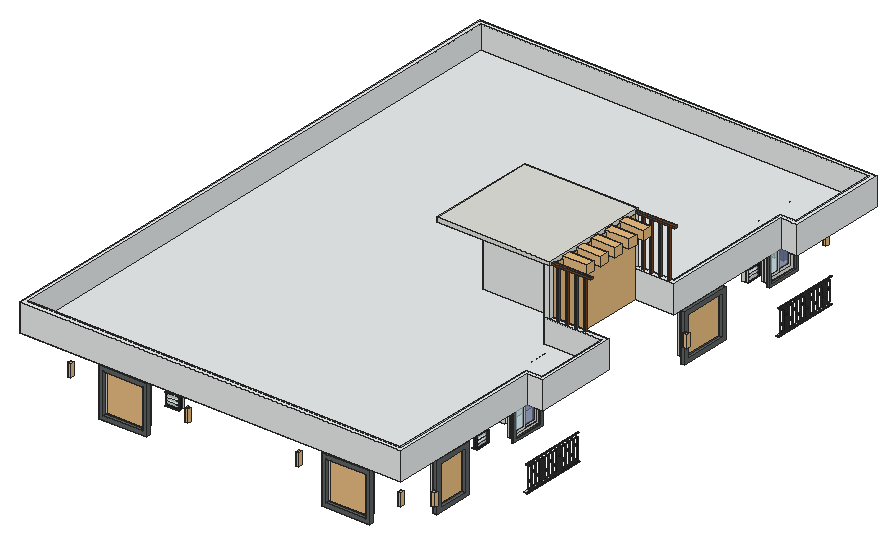
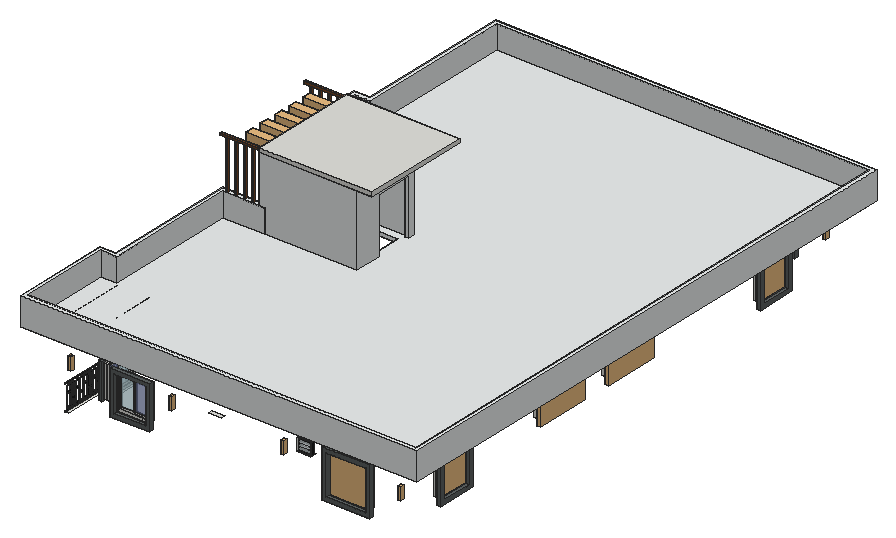
# SketchUp Ruby script. Lengths in inches.
U = 1.inch
M = Sketchup.active_model
def pt(a) = Geom::Point3d.new(a.map { |v| v * U })
def face(e, loops, mat)
  f = e.add_face(loops[0].map { |a| pt(a) })
  loops[1..].each { |l| e.add_face(l.map { |a| pt(a) }).erase! }
  f.material = f.back_material = mat if mat
  f
end
# faces: each face lists its corners as indices into pts; further lists are holes
def faces(e, pts, list, mat = nil) = list.each { |f| face(e, (f[0].is_a?(Array) ? f : [f]).map { |l| l.map { |i| pts[i] } }, mat) }
# xy, xz, yz: faces in a plane at the given z, y or x. An outline is a flat list of corners, or four numbers for a rectangle; further outlines are holes
def ring(l) = l.size == 4 ? [[l[0], l[1]], [l[2], l[1]], [l[2], l[3]], [l[0], l[3]]] : l.each_slice(2).to_a
def flat(e, list, mat, &to3) = list.each { |f| face(e, (f[0].is_a?(Array) ? f : [f]).map { |l| ring(l).map { |u, v| to3.(u, v) } }, mat) }
def xy(e, z, list, mat = nil) = flat(e, list, mat) { |x, y| [x, y, z] }
def xz(e, y, list, mat = nil) = flat(e, list, mat) { |x, z| [x, y, z] }
def yz(e, x, list, mat = nil) = flat(e, list, mat) { |y, z| [x, y, z] }
def lines(e, pts, list) = list.each { |a, b| e.add_line(pt(pts[a]), pt(pts[b])) }
# prism: a flat outline (further loops are holes) pulled along v
def prism(e, loops, v, mat = nil)
  f = face(e, loops, mat); d = Geom::Vector3d.new(v.map { |x| x * U })
  f.pushpull(f.normal.samedirection?(d) ? d.length : -d.length)
end
def box(e, o, s, mat = nil) = prism(e, [[o, [o[0] + s[0], o[1], o[2]], [o[0] + s[0], o[1] + s[1], o[2]], [o[0], o[1] + s[1], o[2]]]], [0, 0, s[2]], mat)
def at(x, y, z, deg = 0) = Geom::Transformation.translation(pt([x, y, z])) * Geom::Transformation.rotation(ORIGIN, Z_AXIS, deg.degrees)
def axes(o, x, y, z) = Geom::Transformation.new([*x, 0, *y, 0, *z, 0, *pt(o).to_a, 1])
def part(name) = M.definitions.add(name)
# library, detail: a bought-in or finely detailed component or shape, given as its bounding box
def library(name, o, s) = part(name).tap { |d| box(d.entities, o, s) }
def detail(e, o, s) = box(e.add_group.entities, o, s)
def put(e, d, t, mat = nil) = e.add_instance(d, t).tap { |i| i.material = mat if mat }
def group(e, t, mat = nil) = e.add_group.tap { |g| g.transformation = t; g.material = mat if mat }.entities
root = M.entities
M.materials.add("1487 AP 8286 CHARCOAL SHADOW").color = [94, 99, 99]
M.materials.add("[3P0081_White-City]").color = [235, 238, 238]
M.materials.add("[Color M08]").color = [30, 30, 30]
M.materials.add("[Color_008]1").color = [30, 30, 30]
M.materials.add("[Translucent Glass Safety]").color = [218, 227, 229]
M.materials["[Translucent Glass Safety]"].alpha = 0.5
M.materials.add("[Translucent_Glass_Safety]").color = [204, 235, 244]
M.materials["[Translucent_Glass_Safety]"].alpha = 0.5
M.materials.add("[Translucent_Glass_Sky_Reflection]").color = [125, 138, 183]
M.materials["[Translucent_Glass_Sky_Reflection]"].alpha = 0.52
M.materials.add("[Wood Veneer 01]").color = [120, 70, 37]
c1 = library("porta 4",[0.2,-5.42,1.33],[46.55,4.72,83.21])
c2 = part("Group\#70")
prism(c2.entities,[[[4.13,0,3.9375],[7.875,0,3.9375],[7.875,0,13.78],[4.13,0,13.78],[4.13,0,15.75],[7.875,0,15.75],[7.875,0,35.43],[4.13,0,35.43],[4.13,0,39.37],[3.74,0,39.37],[3.74,0,35.43],[0,0,35.43],[0,0,15.75],[3.74,0,15.75],[3.74,0,13.78],[0,0,13.78],[0,0,3.9375],[3.74,0,3.9375],[3.74,0,0],[4.13,0,0]],[[0.39,0,16.14],[0.39,0,35.04],[7.48,0,35.04],[7.48,0,16.14]],[[7.48,0,4.33],[0.39,0,4.33],[0.39,0,13.39],[7.48,0,13.39]]],[0,0.39,0],"[Color M08]")
c3 = part("Group\#69")
prism(c3.entities,[[[3.74,0,35.43],[0,0,35.43],[0,0,25.59],[3.74,0,25.59],[3.74,0,23.62],[0,0,23.62],[0,0,3.9375],[3.74,0,3.9375],[3.74,0,0],[4.13,0,0],[4.13,0,3.9375],[7.875,0,3.9375],[7.875,0,23.62],[4.13,0,23.62],[4.13,0,25.59],[7.875,0,25.59],[7.875,0,35.43],[4.13,0,35.43],[4.13,0,39.37],[3.74,0,39.37]],[[7.48,0,23.23],[7.48,0,4.33],[0.39,0,4.33],[0.39,0,23.23]],[[0.39,0,35.04],[7.48,0,35.04],[7.48,0,25.98],[0.39,0,25.98]]],[0,0.39,0],"[Color M08]")
c4 = part("Group\#71")
put(c4.entities,c2,at(0,0,0))
put(c4.entities,c3,at(9.84,0,0))
c5 = part("Group\#79")
g1 = group(c5.entities,at(0,0,0))
box(g1,[0,-2.09,0],[1.97,122.29,0.79],"[Color M08]")
put(c5.entities,c4,axes([0.79,40.35,0.79],[0,1,0],[1,0,0],[0,0,1]))
put(c5.entities,c4,axes([0.79,79.72,0.79],[0,1,0],[1,0,0],[0,0,1]))
put(c5.entities,c4,axes([0.79,60.04,0.79],[0,1,0],[1,0,0],[0,0,1]))
put(c5.entities,c4,axes([0.79,99.41,0.79],[0,1,0],[1,0,0],[0,0,1]))
g2 = group(c5.entities,at(0,0,40.16))
box(g2,[0,-2.09,0],[1.97,122.29,0.79],"[Color M08]")
put(c5.entities,c4,axes([0.79,20.67,0.79],[0,1,0],[1,0,0],[0,0,1]))
put(c5.entities,c4,axes([0.79,0.98,0.79],[0,1,0],[1,0,0],[0,0,1]))
c6 = part("14")
prism(c6.entities,[[[0,60,66],[0,0,66],[0,0,0],[0,60,0]],[[0,54,6],[0,6,6],[0,6,60],[0,54,60]]],[-6,0,0])
c7 = library("15",[-6,0,0],[6,84,66])
c8 = part("17")
prism(c8.entities,[[[0,0,0],[0,0,72],[72,0,72],[72,0,0]],[[6,0,6],[66,0,6],[66,0,66],[6,0,66]]],[0,-6,0])
c9 = library("Group\#98",[0,-5.45,0],[91.05,108.7,8])
c10 = part("Two-panel window")
xy(c10.entities,0,[[0,0,4.33,55.51]])
xy(c10.entities,2.76,[[0,2.76,2,2.76,2,27.76,0.82,27.76,0.82,52.76,0,52.76],[3.15,2.76,4.33,2.76,4.33,52.76,2.36,52.76,2.36,27.76,3.15,27.76],[0.82,27.76,2.36,52.76]])
xy(c10.entities,4.72,[[2,4.72,2.4,26.38],[2.76,4.72,3.15,26.38],[0.82,29.13,1.22,50.79],[1.97,29.13,2.36,50.79]])
xy(c10.entities,36.61,[[2,4.72,2.4,26.38],[2.76,4.72,3.15,26.38],[0.82,29.13,1.22,50.79],[1.97,29.13,2.36,50.79]])
xy(c10.entities,38.58,[[0,2.76,2,27.76],[3.15,2.76,4.33,27.76],[0,27.76,0.82,52.76],[0.82,27.76,2.36,52.76],[2.36,27.76,4.33,52.76]])
xy(c10.entities,41.34,[[0,0,4.33,55.51]])
xz(c10.entities,0,[[0,0,4.33,41.34]])
xz(c10.entities,2.76,[[0,2.76,2,38.58],[3.15,2.76,4.33,38.58]])
xz(c10.entities,4.72,[[2,4.72,2.4,36.61],[2.76,4.72,3.15,36.61]])
xz(c10.entities,26.38,[[2,4.72,2.4,36.61],[2.76,4.72,3.15,36.61]])
xz(c10.entities,27.76,[[0.82,2.76,2,38.58],[2,2.76,2.36,38.58],[2.36,2.76,3.15,38.58]])
xz(c10.entities,29.13,[[0.82,4.72,1.22,36.61],[1.97,4.72,2.36,36.61]])
xz(c10.entities,50.79,[[0.82,4.72,1.22,36.61],[1.97,4.72,2.36,36.61]])
xz(c10.entities,52.76,[[0,2.76,0.82,38.58],[0.82,2.76,2.36,38.58],[2.36,2.76,4.33,38.58]])
xz(c10.entities,55.51,[[0,0,4.33,41.34]])
yz(c10.entities,0,[[[0,0,55.51,41.34],[2.76,2.76,52.76,38.58]]])
yz(c10.entities,0.82,[[[27.76,2.76,52.76,38.58],[29.13,4.72,50.79,36.61]]])
yz(c10.entities,1.22,[[29.13,4.72,50.79,36.61]],"[Translucent_Glass_Sky_Reflection]")
yz(c10.entities,1.97,[[29.13,4.72,50.79,36.61]],"[Translucent_Glass_Sky_Reflection]")
yz(c10.entities,2,[[[2.76,2.76,27.76,38.58],[4.72,4.72,26.38,36.61]]])
yz(c10.entities,2.36,[[[27.76,2.76,52.76,38.58],[29.13,4.72,50.79,36.61]]])
yz(c10.entities,2.4,[[4.72,4.72,26.38,36.61]],"[Translucent_Glass_Safety]")
yz(c10.entities,2.76,[[4.72,4.72,26.38,36.61]],"[Translucent_Glass_Safety]")
yz(c10.entities,3.15,[[[2.76,2.76,27.76,38.58],[4.72,4.72,26.38,36.61]]])
yz(c10.entities,4.33,[[[0,0,55.51,41.34],[2.76,2.76,52.76,38.58]]])
c11 = library("Group\#50",[0,-5.45,0],[91.05,108.7,8])
c12 = library("Group\#36",[0,-5.45,0],[91.05,108.7,8])
c13 = library("Group\#28",[0.125,0,-2.28],[4,104,84.28])
c14 = library("WALL LIGHT 69",[4.19,4.05,-9.73],[4.61,5.7,19.03])
c15 = part("Group\#40")
box(c15.entities,[0,0.25,0],[21,0.25,6],"[Translucent Glass Safety]")
c16 = part("tingkap keping toilet")
g3 = group(c16.entities,at(-23.5,-2,0),"[Color_008]1")
prism(g3,[[[47,0,57],[22.5,0,57],[22.5,0,41.8],[47,0,41.8]],[[24.5,0,43.3],[24.5,0,55.5],[45.5,0,55.5],[45.5,0,43.3]]],[0,4,0])
g4 = group(c16.entities,at(1,-2,47))
put(g4,c15,axes([0,3.73,3.53],[1,0,0],[0,0.757,0.65342],[0,-0.65342,0.757]))
put(g4,c15,axes([0,3.73,-0.17],[1,0,0],[0,0.757,0.65342],[0,-0.65342,0.757]))
put(g4,c15,axes([0,3.73,-3.87],[1,0,0],[0,0.757,0.65342],[0,-0.65342,0.757]))
c17 = library("Floor panel",[0,13.98,-0.38],[148.62,177.51,16.92])
c18 = library("Group\#130",[0,6,-42],[1.25,152,114])
c19 = library("20",[0,-4.6875,-10.69],[37.375,13.375,13.69])
xy(root,266,[[682.5,564.97,688.5,663.97],[553.5,678.97,562.5,738.97],[679.5,1044.97,685.5,1143.97]])
xy(root,294,[[649.5,897.97,658.5,963.97]])
xy(root,300,[[218,357.97,278,366.97],[554.5,357.97,614.5,366.97],[171,426.87,180,474.87],[652.5,426.87,661.5,474.87],[493.5,600.97,513.5,606.97],
  [622.5,609.97,631.5,657.97],[198,654.97,207,726.97],[198,783.97,207,855.97],[171,1029.97,180,1077.97],[493.5,1080.97,513.5,1086.97],
  [622.5,1089.97,631.5,1137.97],[218,1143.97,278,1152.97],[550.5,1143.97,598.5,1152.97]])
xy(root,342,[[306,357.97,327.5,366.97],[652.5,504.97,661.5,526.53],[382.75,726.97,404.25,735.97],[382.75,774.97,404.25,783.97],[649.5,1017.47,658.5,1038.97],
  [306,1143.97,327.5,1152.97]])
xy(root,348,[[309,453.97,333,459.97],[360,462.97,366,492.97],[507,498.97,539,504.97],[553.5,498.97,583.5,504.97],[622.5,567.97,631.5,597.97],
  [622.5,609.97,631.5,657.97],[321,624.97,357,630.97],[433.5,663.97,472.5,672.97],[363,666.97,369,690.97],[363,819.97,369,843.97],
  [433.5,837.97,472.5,846.97],[321,879.97,357,885.97],[504,978.97,536,984.97],[550.5,978.97,580.5,984.97],[360,1017.47,366,1047.47],
  [622.5,1047.97,631.5,1077.97],[309,1050.97,333,1056.97],[622.5,1089.97,631.5,1137.97]])
xy(root,354,[[386.25,387.97,470.25,396.97],[171,426.87,180,474.87],[198,530.97,207,614.97],[198,654.97,207,726.97],[198,783.97,207,855.97],
  [649.5,897.97,658.5,963.97],[198,903.97,207,987.97],[171,1029.97,180,1077.97],[386.25,1113.97,470.25,1122.97],[550.5,1143.97,598.5,1152.97]])
xy(root,360,[[218,357.97,278,366.97],[306,357.97,327.5,366.97],[554.5,357.97,614.5,366.97],[652.5,426.87,661.5,474.87],[652.5,504.97,661.5,526.53],
  [382.75,726.97,404.25,735.97],[382.75,774.97,404.25,783.97],[649.5,1017.47,658.5,1038.97],[218,1143.97,278,1152.97],[306,1143.97,327.5,1152.97]])
xy(root,390,[[[144,357.97,366,357.97,366,387.97,490.5,387.97,490.5,357.97,688.5,357.97,688.5,408.97,661.5,408.97,661.5,529,688.5,529,688.5,535,661.5,535,661.5,558.97,688.5,558.97,688.5,564.97,631.5,564.97,631.5,663.97,688.5,663.97,688.5,672.97,631.5,672.97,631.5,763.97,622.5,763.97,622.5,753.97,553.5,753.97,553.5,738.97,562.5,738.97,562.5,744.97,622.5,744.97,622.5,672.97,562.5,672.97,562.5,678.97,553.5,678.97,553.5,672.97,430.5,672.97,430.5,837.97,622.5,837.97,622.5,827.97,631.5,827.97,631.5,837.97,685.5,837.97,685.5,888.97,658.5,888.97,658.5,1009,685.5,1009,685.5,1015,658.5,1015,658.5,1038.97,649.5,1038.97,649.5,984.97,544.5,984.97,544.5,1038.97,685.5,1038.97,685.5,1044.97,631.5,1044.97,631.5,1143.97,685.5,1143.97,685.5,1152.97,487.5,1152.97,487.5,1122.97,366,1122.97,366,1152.97,144,1152.97,144,1101.97,171,1101.97,171,1005.97,198,1005.97,198,504.97,171,504.97,171,408.97,144,408.97],[366,396.97,366,504.97,207,504.97,207,624.97,427.5,624.97,427.5,663.97,487.5,663.97,487.5,572.47,421.5,572.47,421.5,537.97,427.5,537.97,427.5,566.47,487.5,566.47,487.5,537.97,493.5,537.97,493.5,663.97,622.5,663.97,622.5,564.97,541.5,564.97,541.5,504.97,490.5,504.97,490.5,396.97],[427.5,846.97,427.5,885.97,207,885.97,207,1005.97,366,1005.97,366,1113.97,487.5,1113.97,487.5,1080.97,493.5,1080.97,493.5,1143.97,622.5,1143.97,622.5,1044.97,487.5,1044.97,487.5,1014.97,493.5,1014.97,493.5,1038.97,538.5,1038.97,538.5,984.97,487.5,984.97,487.5,944.47,427.5,944.47,427.5,972.97,421.5,972.97,421.5,938.47,487.5,938.47,487.5,846.97],[496.5,366.97,496.5,495.97,504.5,495.97,504.5,498.97,617.5,498.97,617.5,495.97,631.5,495.97,631.5,498.97,652.5,498.97,652.5,399.97,679.5,399.97,679.5,366.97],[493.5,846.97,493.5,975.97,501.5,975.97,501.5,978.97,617.5,978.97,617.5,975.97,631.5,975.97,631.5,978.97,649.5,978.97,649.5,879.97,676.5,879.97,676.5,846.97],[207,630.97,207,750.97,372,750.97,372,774.97,421.5,774.97,421.5,735.97,372,735.97,372,750.97,363,750.97,363,630.97],[180,1011.97,180,1110.97,153,1110.97,153,1143.97,300,1143.97,300,1050.97,360,1050.97,360,1014.97,352,1014.97,352,1011.97],[153,366.97,153,399.97,180,399.97,180,498.97,352,498.97,352,495.97,360,495.97,360,459.97,300,459.97,300,366.97],[207,759.97,363,879.97],[547.5,504.97,652.5,558.97],[369,783.97,421.5,879.97],[369,630.97,421.5,726.97],[306,366.97,360,453.97],[306,1056.97,360,1143.97]]])
xz(root,426.87,[[171,300,180,354],[652.5,300,661.5,360]])
xz(root,474.87,[[171,300,180,354],[652.5,300,661.5,360]])
xz(root,526.53,[[652.5,342,661.5,360]])
xz(root,609.97,[[622.5,300,631.5,348]])
xz(root,654.97,[[198,300,207,354]])
xz(root,657.97,[[622.5,300,631.5,348]])
xz(root,678.97,[[553.5,266,562.5,390]])
xz(root,726.97,[[198,300,207,354]])
xz(root,738.97,[[553.5,266,562.5,390]])
xz(root,783.97,[[198,300,207,354]])
xz(root,855.97,[[198,300,207,354]])
xz(root,897.97,[[649.5,294,658.5,354]])
xz(root,963.97,[[649.5,294,658.5,354]])
xz(root,1017.47,[[649.5,342,658.5,360]])
xz(root,1029.97,[[171,300,180,354]])
xz(root,1077.97,[[171,300,180,354]])
xz(root,1089.97,[[622.5,300,631.5,348]])
xz(root,1137.97,[[622.5,300,631.5,348]])
yz(root,218,[[357.97,300,366.97,360],[1143.97,300,1152.97,360]])
yz(root,278,[[357.97,300,366.97,360],[1143.97,300,1152.97,360]])
yz(root,327.5,[[357.97,342,366.97,360],[1143.97,342,1152.97,360]])
yz(root,382.75,[[726.97,342,735.97,360],[774.97,342,783.97,360]])
yz(root,404.25,[[726.97,342,735.97,360],[774.97,342,783.97,360]])
yz(root,550.5,[[1143.97,300,1152.97,354]])
yz(root,554.5,[[357.97,300,366.97,360]])
yz(root,598.5,[[1143.97,300,1152.97,354]])
yz(root,614.5,[[357.97,300,366.97,360]])
put(root,c1,axes([472.67,670.54,264],[-0.83352,0,0],[0,1,0],[0,0,1]))
put(root,c1,axes([472.67,840.41,264],[-0.83352,0,0],[0,-1,0],[0,0,1]))
put(root,c5,axes([687.5,566.66,266],[-1,0,0],[0,0.80958,0],[0,0,0.9525]))
put(root,c5,axes([684.5,1046.66,266],[-1,0,0],[0,0.80958,0],[0,0,0.9525]))
g5 = group(root,at(658.5,891.97,288),"1487 AP 8286 CHARCOAL SHADOW")
prism(g5,[[[0,0,72],[0,78,72],[0,78,0],[0,0,0]],[[0,6,6],[0,72,6],[0,72,66],[0,6,66]]],[6,0,0])
put(root,c6,at(171,1023.97,294),"1487 AP 8286 CHARCOAL SHADOW")
put(root,c6,at(171,420.87,294),"1487 AP 8286 CHARCOAL SHADOW")
put(root,c7,at(198,777.97,294),"1487 AP 8286 CHARCOAL SHADOW")
put(root,c7,at(198,648.97,294),"1487 AP 8286 CHARCOAL SHADOW")
put(root,c8,at(212,357.97,294),"1487 AP 8286 CHARCOAL SHADOW")
put(root,c8,at(548.5,357.97,294),"1487 AP 8286 CHARCOAL SHADOW")
g6 = group(root,at(661.5,420.87,294),"1487 AP 8286 CHARCOAL SHADOW")
prism(g6,[[[0,0,0],[0,0,72],[0,60,72],[0,60,0]],[[0,6,66],[0,6,6],[0,54,6],[0,54,66]]],[6,0,0])
g7 = group(root,at(544.5,1152.97,294),"1487 AP 8286 CHARCOAL SHADOW")
prism(g7,[[[60,0,66],[0,0,66],[0,0,0],[60,0,0]],[[54,0,6],[6,0,6],[6,0,60],[54,0,60]]],[0,6,0])
g8 = group(root,at(212,1152.97,294),"1487 AP 8286 CHARCOAL SHADOW")
prism(g8,[[[0,0,72],[0,0,0],[72,0,0],[72,0,72]],[[66,0,66],[66,0,6],[6,0,6],[6,0,66]]],[0,6,0])
put(root,c9,axes([652.6,963.97,297.01],[0,-0.72488,0],[0,0,0.55196],[0.55,0,0]))
g9 = group(root,at(631.5,604.97,295),"1487 AP 8286 CHARCOAL SHADOW")
prism(g9,[[[0,56,2],[0,2,2],[0,2,56],[0,56,56]],[[0,53,5],[0,53,53],[0,5,53],[0,5,5]]],[3,0,0])
g10 = group(root,at(631.5,1084.97,295),"1487 AP 8286 CHARCOAL SHADOW")
prism(g10,[[[0,56,2],[0,2,2],[0,2,56],[0,56,56]],[[0,53,5],[0,53,53],[0,5,53],[0,5,5]]],[5,0,0])
put(root,c9,axes([655.6,474.87,303.01],[0,-0.52718,0],[0,0,0.55196],[0.55,0,0]))
put(root,c10,axes([625.67,609.97,300],[1,0,0],[0,0.86468,0],[0,0,1.16114]))
put(root,c10,axes([625.67,1089.97,300],[1,0,0],[0,0.86468,0],[0,0,1.16114]))
put(root,c10,axes([598.5,1147.14,300],[0,1,0],[-0.86468,0,0],[0,0,1.30629]))
put(root,c11,axes([554.5,363.875,303.01],[0.65898,0,0],[0,0,0.55196],[0,-0.55,0]))
put(root,c9,axes([218,363.875,303.01],[0.65898,0,0],[0,0,0.55196],[0,-0.55,0]))
put(root,c12,axes([218,1147.07,303.01],[0.65898,0,0],[0,0,0.55196],[0,0.55,0]))
put(root,c13,axes([198.875,654.97,301.46],[1,0,0],[0,0.69231,0],[0,0,0.64074]))
put(root,c13,axes([198.875,855.97,301.46],[1,0,0],[0,-0.69231,0],[0,0,0.64074]))
put(root,c9,axes([176.9,474.87,302.71],[0,-0.52718,0],[0,0,0.49676],[-0.55,0,0]))
put(root,c9,axes([176.9,1029.97,302.71],[0,0.52718,0],[0,0,0.49676],[-0.55,0,0]))
put(root,c14,at(642,709.2,337.375,90))
put(root,c14,at(699.24,377.55,340.64,90))
put(root,c14,at(696.49,856.8,343.25,90))
put(root,c14,at(505.9375,347.23,344.67))
put(root,c14,axes([173.78,346.73,344.67],[-1,0,0],[0,1,0],[0,0,1]))
put(root,c14,axes([350.5625,347.23,344.67],[-1,0,0],[0,1,0],[0,0,1]))
put(root,c14,at(658.9375,347.23,344.67))
put(root,c14,axes([505.9375,1163.72,344.67],[1,0,0],[0,-1,0],[0,0,1]))
put(root,c14,at(173.78,1164.22,344.67,180))
put(root,c14,at(350.5625,1163.72,344.67,180))
put(root,c14,axes([658.9375,1163.72,344.67],[1,0,0],[0,-1,0],[0,0,1]))
put(root,c16,axes([658,525.65,292.5],[0,-0.87972,0],[1,0,0],[0,0,1.18421]))
put(root,c16,axes([403.42,732.47,292.5],[-0.87972,0,0],[0,-1,0],[0,0,1.18421]))
put(root,c16,axes([658,1038.15,292.5],[0,-0.87972,0],[1,0,0],[0,0,1.18421]))
put(root,c16,axes([326.67,361.47,292.5],[-0.87972,0,0],[0,-1,0],[0,0,1.18421]))
put(root,c16,axes([326.67,1149.47,292.5],[-0.87972,0,0],[0,1,0],[0,0,1.18421]))
put(root,c17,axes([496.83,339.97,388.54],[0,0.30278,0],[-0.66754,0,0],[0,0,0.27]))
put(root,c17,axes([493.59,1174.04,388.54],[0,-0.33306,0],[-0.65064,0,0],[0,0,0.27]))
g11 = group(root,at(144,357.97,402),"[3P0081_White-City]")
xy(g11,-12,[[[-27,-36,-27,831,571.99,831,571.99,681,547.99,681,547.99,479,487.5,479,487.5,327,571.99,327,571.99,201,547.99,201,547.99,-36],[349.5,396,478.5,480],[487.5,207,544.75,306],[225,768,340.5,816],[487.5,687,541.75,786],[225,-18,343.5,27]],[[487.5,207,544.75,306],[490.5,210,541.75,303]]])
xy(g11,-9,[[225,-18,343.5,27],[490.5,210,541.75,303],[487.5,687,541.75,786],[225,768,340.5,816]])
xy(g11,-6,[[-21,-30,541.99,-30,541.99,207,565.99,207,565.99,321,478.5,321,478.5,396,349.5,396,349.5,480,478.5,480,478.5,486,541.99,486,541.99,687,565.99,687,565.99,825,-21,825]])
xy(g11,30,[[[-27,-36,547.99,-36,547.99,201,571.99,201,571.99,327,487.5,327,487.5,479,547.99,479,547.99,681,571.99,681,571.99,831,-27,831],[-21,-30,-21,825,565.99,825,565.99,687,541.99,687,541.99,486,478.5,486,478.5,321,565.99,321,565.99,207,541.99,207,541.99,-30]]])
xz(g11,-36,[[-27,-12,547.99,30]])
xz(g11,-30,[[-21,-6,541.99,30]])
xz(g11,-18,[[225,-12,343.5,-9]])
xz(g11,27,[[225,-12,343.5,-9]])
xz(g11,201,[[547.99,-12,571.99,30]])
xz(g11,207,[[541.99,-6,565.99,30]])
xz(g11,210,[[490.5,-12,541.75,-9]])
xz(g11,303,[[490.5,-12,541.75,-9]])
xz(g11,321,[[478.5,-6,565.99,30]])
xz(g11,327,[[487.5,-12,571.99,30]])
xz(g11,396,[[349.5,-12,478.5,-6]])
xz(g11,479,[[487.5,-12,547.99,30]])
xz(g11,480,[[349.5,-12,478.5,-6]])
xz(g11,486,[[478.5,-6,541.99,30]])
xz(g11,681,[[547.99,-12,571.99,30]])
xz(g11,687,[[487.5,-12,541.75,-9],[541.99,-6,565.99,30]])
xz(g11,768,[[225,-12,340.5,-9]])
xz(g11,786,[[487.5,-12,541.75,-9]])
xz(g11,816,[[225,-12,340.5,-9]])
xz(g11,825,[[-21,-6,565.99,30]])
xz(g11,831,[[-27,-12,571.99,30]])
yz(g11,-27,[[-36,-12,831,30]])
yz(g11,-21,[[-30,-6,825,30]])
yz(g11,225,[[-18,-12,27,-9],[768,-12,816,-9]])
yz(g11,340.5,[[768,-12,816,-9]])
yz(g11,343.5,[[-18,-12,27,-9]])
yz(g11,349.5,[[396,-12,480,-6]])
yz(g11,478.5,[[396,-12,396,-6,321,-6,321,30,486,30,486,-6,480,-6,480,-12]])
yz(g11,487.5,[[327,-12,479,30],[687,-12,786,-9]])
yz(g11,490.5,[[210,-12,303,-9]])
yz(g11,541.75,[[210,-12,303,-9],[687,-12,786,-9]])
yz(g11,541.99,[[-30,-6,207,30],[486,-6,687,30]])
yz(g11,547.99,[[-36,-12,201,30],[479,-12,681,30]])
yz(g11,565.99,[[207,-6,321,30],[687,-6,825,30]])
yz(g11,571.99,[[201,-12,327,30],[681,-12,831,30]])
p = [[222,30,-12],[346.5,30,-12],[343.5,765,-12],[222,765,-12]]
lines(g11,p,[[0,1],[2,3]])
put(root,c18,at(631.5,678.97,432))
put(root,c17,axes([634.5,1040.65,390.32],[0.32297,0,0],[0,0.52389,0],[0,0,0.27]))
put(root,c17,axes([637.5,560.65,390.32],[0.32297,0,0],[0,0.52389,0],[0,0,0.27]))
g12 = group(root,at(615.3125,837.97,396))
xy(g12,0,[[-130.8125,-102,-130.8125,-93,-124.8125,-93,-124.8125,-96,7.1875,-96,7.1875,-102],[-130.8125,-36,-130.8125,6,7.1875,6,7.1875,0,-124.8125,0,-124.8125,-36]],"[3P0081_White-City]")
xy(g12,36,[[7.1875,-159,16.1875,6]],"[3P0081_White-City]")
xy(g12,84,[[-130.8125,-93,-124.8125,-36]],"[3P0081_White-City]")
xy(g12,108,[[[7.1875,-159,16.1875,-159,16.1875,6,-130.8125,6,-130.8125,-102,7.1875,-102],[-124.8125,-96,7.1875,0]]],"[3P0081_White-City]")
xz(g12,-159,[[7.1875,36,16.1875,108]],"[3P0081_White-City]")
xz(g12,-102,[[-130.8125,0,7.1875,108]],"[3P0081_White-City]")
xz(g12,-96,[[-124.8125,0,7.1875,108]],"[3P0081_White-City]")
xz(g12,-93,[[-130.8125,0,-124.8125,84]],"[3P0081_White-City]")
xz(g12,-36,[[-130.8125,0,-124.8125,84]],"[3P0081_White-City]")
xz(g12,0,[[-124.8125,0,7.1875,108]],"[3P0081_White-City]")
xz(g12,6,[[-130.8125,0,-130.8125,108,16.1875,108,16.1875,36,7.1875,36,7.1875,0]],"[3P0081_White-City]")
yz(g12,-130.8125,[[-102,0,-102,108,6,108,6,0,-36,0,-36,84,-93,84,-93,0]],"[3P0081_White-City]")
yz(g12,-124.8125,[[-36,0,0,0,0,108,-96,108,-96,84,-36,84],[-96,0,-93,84]],"[3P0081_White-City]")
yz(g12,7.1875,[[-102,0,-96,36],[0,0,6,36],[-159,36,-102,108],[-96,36,0,108]],"[3P0081_White-City]")
yz(g12,16.1875,[[-159,36,6,108]],"[3P0081_White-City]")
g13 = group(root,at(631.5,838.97,505.5),"[Wood Veneer 01]")
xy(g13,-73.5,[[9,1,12,3],[22.16,1,25.16,3],[35.33,1,38.33,3],[48.49,1,51.49,3]])
xy(g13,0,[[[0,0,60.49,4],[9,1,12,3],[22.16,1,25.16,3],[35.33,1,38.33,3],[48.49,1,51.49,3]]])
xy(g13,3,[[0,0,60.49,4]])
xz(g13,0,[[0,0,60.49,3]])
xz(g13,1,[[9,-73.5,12,0],[22.16,-73.5,25.16,0],[35.33,-73.5,38.33,0],[48.49,-73.5,51.49,0]])
xz(g13,3,[[9,-73.5,12,0],[22.16,-73.5,25.16,0],[35.33,-73.5,38.33,0],[48.49,-73.5,51.49,0]])
xz(g13,4,[[0,0,60.49,3]])
yz(g13,0,[[0,0,4,3]])
yz(g13,9,[[1,-73.5,3,0]])
yz(g13,12,[[1,-73.5,3,0]])
yz(g13,22.16,[[1,-73.5,3,0]])
yz(g13,25.16,[[1,-73.5,3,0]])
yz(g13,35.33,[[1,-73.5,3,0]])
yz(g13,38.33,[[1,-73.5,3,0]])
yz(g13,48.49,[[1,-73.5,3,0]])
yz(g13,51.49,[[1,-73.5,3,0]])
yz(g13,60.49,[[0,0,4,3]])
g14 = group(root,at(631.5,683.97,505.5),"[Wood Veneer 01]")
xy(g14,-73.5,[[9,-3,12,-1],[22.16,-3,25.16,-1],[35.33,-3,38.33,-1],[48.49,-3,51.49,-1]])
xy(g14,0,[[[0,-4,60.49,0],[9,-3,12,-1],[22.16,-3,25.16,-1],[35.33,-3,38.33,-1],[48.49,-3,51.49,-1]]])
xy(g14,3,[[0,-4,60.49,0]])
xz(g14,-4,[[0,0,60.49,3]])
xz(g14,-3,[[9,-73.5,12,0],[22.16,-73.5,25.16,0],[35.33,-73.5,38.33,0],[48.49,-73.5,51.49,0]])
xz(g14,-1,[[9,-73.5,12,0],[22.16,-73.5,25.16,0],[35.33,-73.5,38.33,0],[48.49,-73.5,51.49,0]])
xz(g14,0,[[0,0,60.49,3]])
yz(g14,0,[[-4,0,0,3]])
yz(g14,9,[[-3,-73.5,-1,0]])
yz(g14,12,[[-3,-73.5,-1,0]])
yz(g14,22.16,[[-3,-73.5,-1,0]])
yz(g14,25.16,[[-3,-73.5,-1,0]])
yz(g14,35.33,[[-3,-73.5,-1,0]])
yz(g14,38.33,[[-3,-73.5,-1,0]])
yz(g14,48.49,[[-3,-73.5,-1,0]])
yz(g14,51.49,[[-3,-73.5,-1,0]])
yz(g14,60.49,[[-4,0,0,3]])
put(root,c19,at(631.5,705.81,505.5),"[Wood Veneer 01]")
put(root,c19,at(631.5,732.64,505.5),"[Wood Veneer 01]")
put(root,c19,at(631.5,759.47,505.5),"[Wood Veneer 01]")
put(root,c19,at(631.5,786.31,505.5),"[Wood Veneer 01]")
put(root,c19,at(631.5,813.14,505.5),"[Wood Veneer 01]")
g15 = group(root,at(484.5,678.97,504))
box(g15,[-24,0,0],[171,165,6])
